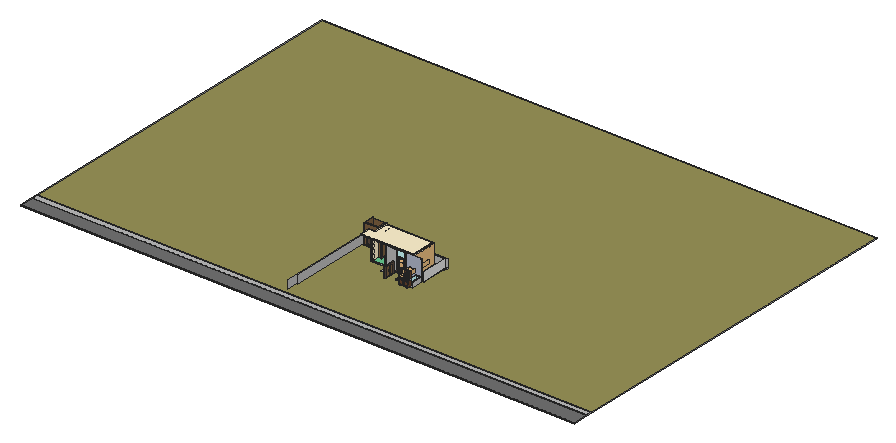
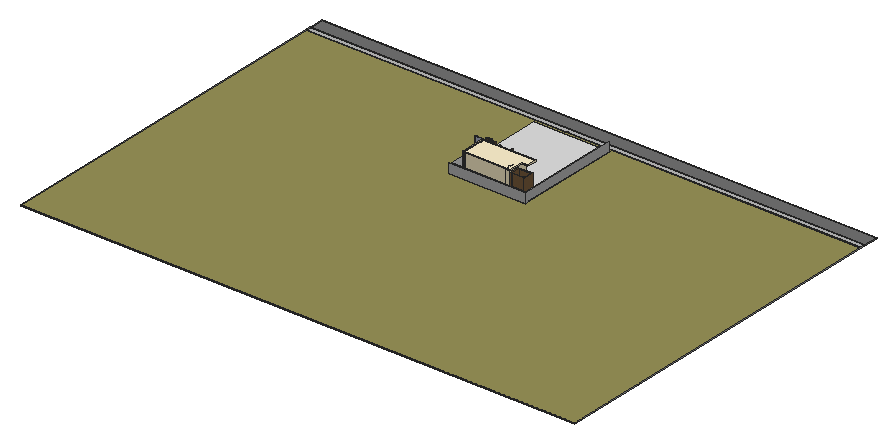
# SketchUp Ruby script. Lengths in inches.
U = 1.inch
M = Sketchup.active_model
def pt(a) = Geom::Point3d.new(a.map { |v| v * U })
def face(e, loops, mat)
  f = e.add_face(loops[0].map { |a| pt(a) })
  loops[1..].each { |l| e.add_face(l.map { |a| pt(a) }).erase! }
  f.material = f.back_material = mat if mat
  f
end
# faces: each face lists its corners as indices into pts; further lists are holes
def faces(e, pts, list, mat = nil) = list.each { |f| face(e, (f[0].is_a?(Array) ? f : [f]).map { |l| l.map { |i| pts[i] } }, mat) }
# xy, xz, yz: faces in a plane at the given z, y or x. An outline is a flat list of corners, or four numbers for a rectangle; further outlines are holes
def ring(l) = l.size == 4 ? [[l[0], l[1]], [l[2], l[1]], [l[2], l[3]], [l[0], l[3]]] : l.each_slice(2).to_a
def flat(e, list, mat, &to3) = list.each { |f| face(e, (f[0].is_a?(Array) ? f : [f]).map { |l| ring(l).map { |u, v| to3.(u, v) } }, mat) }
def xy(e, z, list, mat = nil) = flat(e, list, mat) { |x, y| [x, y, z] }
def xz(e, y, list, mat = nil) = flat(e, list, mat) { |x, z| [x, y, z] }
def yz(e, x, list, mat = nil) = flat(e, list, mat) { |y, z| [x, y, z] }
def lines(e, pts, list) = list.each { |a, b| e.add_line(pt(pts[a]), pt(pts[b])) }
# prism: a flat outline (further loops are holes) pulled along v
def prism(e, loops, v, mat = nil)
  f = face(e, loops, mat); d = Geom::Vector3d.new(v.map { |x| x * U })
  f.pushpull(f.normal.samedirection?(d) ? d.length : -d.length)
end
def box(e, o, s, mat = nil) = prism(e, [[o, [o[0] + s[0], o[1], o[2]], [o[0] + s[0], o[1] + s[1], o[2]], [o[0], o[1] + s[1], o[2]]]], [0, 0, s[2]], mat)
def at(x, y, z, deg = 0) = Geom::Transformation.translation(pt([x, y, z])) * Geom::Transformation.rotation(ORIGIN, Z_AXIS, deg.degrees)
def axes(o, x, y, z) = Geom::Transformation.new([*x, 0, *y, 0, *z, 0, *pt(o).to_a, 1])
def part(name) = M.definitions.add(name)
# library, detail: a bought-in or finely detailed component or shape, given as its bounding box
def library(name, o, s) = part(name).tap { |d| box(d.entities, o, s) }
def detail(e, o, s) = box(e.add_group.entities, o, s)
def put(e, d, t, mat = nil) = e.add_instance(d, t).tap { |i| i.material = mat if mat }
def group(e, t, mat = nil) = e.add_group.tap { |g| g.transformation = t; g.material = mat if mat }.entities
root = M.entities
M.materials.add("Brick_Stack_Bond_2K1").color = [104, 201, 144]
M.materials.add("Brick_Stack_Bond_2K2").color = [186, 186, 186]
M.materials.add("C02_Golden_Beige").color = [255, 205, 155]
M.materials.add("D01_Frost_White").color = [255, 242, 206]
M.materials.add("E03_Spring_Dew").color = [255, 255, 101]
M.materials.add("Glass_Sky Reflection_1").color = [126, 138, 183]
M.materials["Glass_Sky Reflection_1"].alpha = 0.25
M.materials.add("H01_Misty_Ice1").color = [204, 255, 255]
M.materials.add("M00_Soft_Cloud").color = [255, 255, 255]
M.materials.add("M01_Silver_Fog").color = [224, 224, 224]
M.materials.add("M02_Ash_Whisper").color = [196, 196, 196]
M.materials.add("M03_Pewter_Shine").color = [168, 168, 168]
M.materials.add("M05_Graphite_Haze").color = [114, 114, 114]
M.materials.add("M09_Shadow_Night").color = [0, 0, 0]
M.materials.add("Marble_03_1K").color = [175, 182, 201]
M.materials.add("Marble_07_1K").color = [36, 34, 36]
M.materials.add("Metal_06_1K").color = [238, 236, 231]
M.materials.add("Plaster_04_1K").color = [106, 98, 87]
M.materials.add("Plywood_01_1K").color = [125, 96, 64]
M.materials.add("Soil_04_1K").color = [167, 182, 67]
M.materials.add("Soil_04_1K1").color = [152, 146, 88]
M.materials.add("Wood_Floor_01_1K1").color = [146, 111, 76]
M.materials.add("Wood_Floor_12_1K").color = [92, 75, 65]
M.materials.add("Wood_Veneer_15_1K").color = [103, 69, 45]
c1 = part("Group\#174")
box(c1.entities,[0,0,0],[1.8125,10.875,0.375],"Metal_06_1K")
c2 = part("Shower Cabin 003")
xy(c2.entities,0,[[-0.1,-35.53,-0.1,-0.1,35.33,-35.53],[35.33,-35.53,-0.1,-0.1,35.33,-0.1]])
xy(c2.entities,0.39,[[2.26,-33.17,32.97,-2.46,2.26,-2.46],[2.26,-33.17,32.97,-33.17,32.97,-2.46]])
xy(c2.entities,1.18,[[-0.1,-35.53,1.48,-1.67,-0.1,-0.1],[-0.1,-35.53,1.48,-33.96,1.48,-1.67],[-0.1,-35.53,35.33,-35.53,1.48,-33.96],[35.33,-35.53,33.76,-33.96,1.48,-33.96],[35.33,-35.53,35.33,-0.1,33.76,-33.96],
  [33.76,-33.96,35.33,-0.1,33.76,-1.67],[1.48,-1.67,33.76,-1.67,-0.1,-0.1],[33.76,-1.67,35.33,-0.1,-0.1,-0.1]])
xz(c2.entities,-35.53,[[-0.1,0,35.33,0,35.33,1.18],[-0.1,0,35.33,1.18,-0.1,1.18]])
xz(c2.entities,-0.1,[[-0.1,0,-0.1,1.18,35.33,0],[35.33,0,-0.1,1.18,35.33,1.18]])
yz(c2.entities,-0.1,[[-0.1,0,-35.53,1.18,-0.1,1.18],[-35.53,0,-35.53,1.18,-0.1,0]])
yz(c2.entities,35.33,[[-35.53,0,-0.1,0,-0.1,1.18],[-35.53,0,-0.1,1.18,-35.53,1.18]])
p = [[1.48,-33.96,1.18],[2.26,-2.46,0.39],[1.48,-1.67,1.18],[33.76,-33.96,1.18],[2.26,-33.17,0.39],[32.97,-33.17,0.39],
  [33.76,-1.67,1.18],[32.97,-2.46,0.39]]
faces(c2.entities,p,[[0,1,2],[3,4,0],[0,4,1],[3,5,4],[6,5,3],[6,7,5],[2,7,6],[2,1,7]])
c3 = library("Hospital Sink 001",[-20.625,-17.4375,27.15],[31.24,200.7,22.96])
c4 = library("Group\#265",[0,0,0],[16.41,13,26.86])
c5 = library("Group\#200",[-159,9,0],[183,135,46])
c6 = library("Group\#210",[-7.75,0,-2.45],[16.75,48,50.51])
c7 = library("Group\#232",[-0.03,0,0],[10.08,153,132])
c8 = library("Group\#259",[0,0,0],[16.41,13,26.86])
xy(root,6,[[1567.75,149.6875,2047.75,798.625],[1567.75,798.625,1567.75,815.6875,2047.75,815.6875,2047.75,798.625,2044.5625,798.625,2044.5625,806.6875,1574.3125,806.6875,1574.3125,798.625]],"M01_Silver_Fog")
xy(root,12,[[1810.75,590.6875,1876.75,626.6875],[1926.75,626.6875,1939.75,635.6875],[1712.6875,635.6875,1721.6875,635.6875,1721.6875,779.6875,1977.9375,779.6875,1977.9375,635.6875,1986.9375,635.6875,1986.9375,788.6875,1712.6875,788.6875],[1721.6875,635.6875,1977.9375,779.6875]],"Brick_Stack_Bond_2K2")
xy(root,12,[[1886.75,626.6875,1926.75,635.6875]],"H01_Misty_Ice1")
xy(root,12,[[2044.5625,635.6875,2047.75,798.625],[1584.5,798.625,1674.5,806.6875]],"M01_Silver_Fog")
xy(root,12,[[1712.6875,635.6875,1986.9375,788.6875]],"M02_Ash_Whisper")
xy(root,12,[[1574.3125,798.625,1584.5,806.6875],[1674.5,798.625,2044.5625,806.6875]],"Soil_04_1K")
xy(root,18,[[1712.6875,635.6875,1942.625,635.6875,1942.625,671,1977.9375,671,1977.9375,635.6875,1986.9375,635.6875,1986.9375,788.6875,1712.6875,788.6875]],"Brick_Stack_Bond_2K1")
xy(root,18,[[1876.75,602.25,1882.75,626.6875],[1590.5,746.6875,1668.5,802.6875]],"Brick_Stack_Bond_2K2")
xy(root,18,[[1882.75,625.625,1886.75,626.6875],[1926.75,625.625,1930.75,626.6875],[1584.5,740.6875,1584.5,806.6875,1674.5,806.6875,1674.5,740.6875,1635.0625,740.6875,1635.0625,746.6875,1668.5,746.6875,1668.5,802.6875,1590.5,802.6875,1590.5,746.6875,1599.0625,746.6875,1599.0625,740.6875],[1599.0625,740.6875,1635.0625,746.6875]],"Plywood_01_1K")
xy(root,21.375,[[1942.625,635.6875,1977.9375,671]],"M02_Ash_Whisper")
xy(root,71.8125,[[1942.625,635.6875,1977.9375,671]],"M02_Ash_Whisper")
xy(root,73.25,[[1942.625,635.6875,1977.9375,671]],"M02_Ash_Whisper")
xy(root,99.75,[[1942.625,635.6875,1977.9375,671]],"M02_Ash_Whisper")
xy(root,100.8125,[[1942.625,635.6875,1977.9375,671]],"M00_Soft_Cloud")
xz(root,602.25,[[1876.75,18,1882.75,82.875]],"H01_Misty_Ice1")
xz(root,625.625,[[1882.75,18,1886.75,18,1886.75,99,1926.75,99,1926.75,18,1930.75,18,1930.75,103,1882.75,103]],"Plywood_01_1K")
xz(root,626.6875,[[1810.75,12,1876.75,139],[1926.75,12,1930.75,18],[1876.75,18,1882.75,144],[1882.75,18,1886.75,23],[1926.75,18,1930.75,103]],"Brick_Stack_Bond_2K2")
xz(root,626.6875,[[1876.75,12,1886.75,18],[1930.75,12,1939.75,12,1939.75,139,1882.75,139,1882.75,103,1930.75,103]],"H01_Misty_Ice1")
xz(root,635.6875,[[1986.9375,12,2044.5625,18],[2044.5625,12,2047.75,18]],"D01_Frost_White")
xz(root,635.6875,[[1810.75,12,1810.75,139,1939.75,139,1939.75,12,1926.75,12,1926.75,99,1886.75,99,1886.75,12],[1939.75,12,1977.9375,18],[1977.9375,12,1986.9375,18]],"H01_Misty_Ice1")
xz(root,635.6875,[[1942.625,21.375,1977.9375,71.8125],[1942.625,73.25,1977.9375,99.75]],"M00_Soft_Cloud")
xz(root,635.6875,[[2044.5625,18,2047.75,66]],"M01_Silver_Fog")
xz(root,635.6875,[[1712.6875,12,1986.9375,12,1986.9375,18,1977.9375,18,1977.9375,21.375,1942.625,21.375,1942.625,18,1712.6875,18],[1942.625,71.8125,1977.9375,73.25],[1942.625,99.75,1977.9375,100.8125]],"M02_Ash_Whisper")
xz(root,671,[[1942.625,21.375,1977.9375,71.8125],[1942.625,73.25,1977.9375,99.75]],"M00_Soft_Cloud")
xz(root,671,[[1942.625,18,1977.9375,21.375],[1942.625,71.8125,1977.9375,73.25],[1942.625,99.75,1977.9375,100.8125]],"M02_Ash_Whisper")
xz(root,740.6875,[[1584.5,12,1674.5,18],[1584.5,18,1599.0625,18,1599.0625,102,1635.0625,102,1635.0625,18,1674.5,18,1674.5,139,1584.5,139]],"Plywood_01_1K")
xz(root,746.6875,[[1590.5,18,1590.5,139,1668.5,139,1668.5,18,1635.0625,18,1635.0625,102,1599.0625,102,1599.0625,18]],"Plywood_01_1K")
xz(root,788.6875,[[1712.6875,12,1986.9375,18]],"M02_Ash_Whisper")
xz(root,798.625,[[1567.75,6,1574.3125,12],[1574.3125,6,2044.5625,12],[2044.5625,6,2047.75,12]],"M01_Silver_Fog")
xz(root,802.6875,[[1590.5,18,1668.5,139]],"Plywood_01_1K")
xz(root,806.6875,[[1674.5,12,2044.5625,66]],"Brick_Stack_Bond_2K2")
xz(root,806.6875,[[1574.3125,6,1584.5,12],[1584.5,6,1674.5,12],[1674.5,6,2044.5625,12]],"M01_Silver_Fog")
xz(root,806.6875,[[1574.3125,12,1584.5,66]],"M03_Pewter_Shine")
xz(root,806.6875,[[1584.5,12,1674.5,18],[1584.5,18,1674.5,66]],"Plywood_01_1K")
xz(root,815.6875,[[2047.75,0,2053.75,12],[1567.75,6,1567.75,66,2053.75,66,2053.75,12,2047.75,12,2047.75,6]],"Brick_Stack_Bond_2K2")
yz(root,1567.75,[[798.625,6,798.625,12,155.6875,12,155.6875,66,815.6875,66,815.6875,6]],"Brick_Stack_Bond_2K2")
yz(root,1574.3125,[[224.6875,12,806.6875,66]],"Brick_Stack_Bond_2K2")
yz(root,1574.3125,[[798.625,6,806.6875,12]],"M01_Silver_Fog")
yz(root,1584.5,[[740.6875,12,806.6875,18],[740.6875,18,806.6875,139]],"Plywood_01_1K")
yz(root,1590.5,[[746.6875,18,802.6875,139]],"Plywood_01_1K")
yz(root,1599.0625,[[740.6875,18,746.6875,102]],"Plywood_01_1K")
yz(root,1635.0625,[[740.6875,18,746.6875,102]],"Plywood_01_1K")
yz(root,1668.5,[[746.6875,18,802.6875,139]],"Plywood_01_1K")
yz(root,1674.5,[[740.6875,12,806.6875,18],[740.6875,18,806.6875,139]],"Plywood_01_1K")
yz(root,1712.6875,[[635.6875,12,788.6875,18]],"M02_Ash_Whisper")
yz(root,1810.75,[[626.6875,12,635.6875,139]],"Brick_Stack_Bond_2K2")
yz(root,1882.75,[[625.625,18,626.6875,23]],"Brick_Stack_Bond_2K2")
yz(root,1882.75,[[602.25,18,625.625,23]],"Wood_Floor_12_1K")
yz(root,1886.75,[[626.6875,12,635.6875,99]],"H01_Misty_Ice1")
yz(root,1886.75,[[625.625,18,626.6875,99]],"Plywood_01_1K")
yz(root,1926.75,[[626.6875,12,635.6875,99]],"H01_Misty_Ice1")
yz(root,1926.75,[[625.625,18,626.6875,99]],"Plywood_01_1K")
yz(root,1930.75,[[625.625,18,626.6875,103]],"Plywood_01_1K")
yz(root,1939.75,[[626.6875,12,635.6875,18]],"Brick_Stack_Bond_2K2")
yz(root,1939.75,[[626.6875,18,635.6875,139]],"H01_Misty_Ice1")
yz(root,1939.75,[[569.6875,12,626.6875,18]],"Marble_03_1K")
yz(root,1942.625,[[635.6875,21.375,671,71.8125],[635.6875,73.25,671,99.75]],"M00_Soft_Cloud")
yz(root,1942.625,[[635.6875,18,671,21.375],[635.6875,71.8125,671,73.25],[635.6875,99.75,671,100.8125]],"M02_Ash_Whisper")
yz(root,1977.9375,[[635.6875,18,671,21.375],[635.6875,21.375,671,71.8125]],"Brick_Stack_Bond_2K1")
yz(root,1977.9375,[[635.6875,71.8125,671,73.25],[635.6875,73.25,671,99.75],[635.6875,99.75,671,100.8125]],"M02_Ash_Whisper")
yz(root,1986.9375,[[635.6875,12,788.6875,18]],"M02_Ash_Whisper")
yz(root,2044.5625,[[798.625,6,806.6875,12],[635.6875,12,806.6875,66]],"M01_Silver_Fog")
p = [[1926.75,626.6875,18],[1886.75,626.6875,18]]
lines(root,p,[[0,1]])
g1 = group(root,at(1876.75,533.5,18),"Brick_Stack_Bond_2K2")
xy(g1,0,[[0,0,6,68.75]],"Wood_Floor_12_1K")
xy(g1,0.75,[[0,5.4375,4.5,34.21],[0,35.41,4.5,64.1875]])
xy(g1,0.75,[[4.5,5.4375,6,34.21],[0,34.21,6,35.41],[4.5,35.41,6,64.1875]],"Wood_Floor_12_1K")
xy(g1,59.875,[[0,5,4.5,34.21],[0,35.41,4.5,63.75]])
xy(g1,59.875,[[4.5,5,6,34.21],[0,34.21,6,35.41],[4.5,35.41,6,63.75]],"Wood_Floor_12_1K")
xy(g1,64.875,[[0,0,6,68.75]],"Wood_Floor_12_1K")
xz(g1,0,[[0,0,6,64.875]],"Wood_Floor_12_1K")
xz(g1,34.21,[[4.5,0.75,6,59.875]],"Wood_Floor_12_1K")
xz(g1,35.41,[[4.5,0.75,6,59.875]],"Wood_Floor_12_1K")
xz(g1,68.75,[[0,0,6,64.875]],"Wood_Floor_12_1K")
yz(g1,0,[[[0,0,68.75,64.875],[5.4375,0.75,64.1875,0.75,63.75,59.875,5,59.875]]],"Wood_Floor_12_1K")
yz(g1,4.5,[[5.4375,0.75,34.21,0.75,34.21,59.875,5,59.875],[35.41,0.75,64.1875,0.75,63.75,59.875,35.41,59.875]],"Plywood_01_1K")
yz(g1,6,[[[0,0,68.75,64.875],[5.4375,0.75,5,59.875,63.75,59.875,64.1875,0.75]],[34.21,0.75,35.41,59.875]],"Wood_Floor_12_1K")
p = [[0,5.4375,0.75],[0,5,59.875],[4.5,5,59.875],[4.5,5.4375,0.75],[6,5.4375,0.75],[6,5,59.875],
  [0,63.75,59.875],[0,64.1875,0.75],[4.5,64.1875,0.75],[4.5,63.75,59.875],[6,63.75,59.875],[6,64.1875,0.75]]
faces(g1,p,[[0,1,2,3],[6,7,8,9]])
faces(g1,p,[[4,3,2,5],[10,9,8,11]],"Wood_Floor_12_1K")
put(g1,c1,axes([4.5,28.44,28.59],[0,1,0],[0,0,1],[1,0,0]))
put(g1,c1,axes([4.5,38.94,28.59],[0,1,0],[0,0,1],[1,0,0]))
g2 = group(root,at(2002.95,558.2,18),"M02_Ash_Whisper")
p = [[35.375,-0.32,18.93],[0.01,-0.33,18.93],[0.01,0.17,-9.625],[35.375,0.17,-9.625],[0,67.67,20.12],[0,68.17,-8.44],
  [35.37,67.68,20.12],[35.37,68.17,-8.44],[2.68,64.99,20.07],[2.69,2.35,18.98],[2.69,2.68,0.17],[2.68,65.32,1.26],
  [32.69,2.36,18.98],[32.69,2.68,0.17],[32.68,64.99,20.07],[32.68,65.32,1.26]]
faces(g2,p,[[0,1,2,3],[1,4,5,2],[6,0,3,7],[7,3,2,5],[4,6,7,5],[[0,6,4,1],[9,8,14,12]]])
faces(g2,p,[[8,9,10,11],[9,12,13,10],[12,14,15,13],[11,10,13,15],[14,8,11,15]],"H01_Misty_Ice1")
put(root,c2,axes([1932.45,626.78,18],[1.99615,0,0],[0,1.9303,0],[0,0,1]),"M02_Ash_Whisper")
g3 = group(root,at(1939.75,626.6875,18),"M02_Ash_Whisper")
box(g3,[-8.0625,-0.5,0],[107.0625,0.5,126],"Marble_03_1K")
g4 = group(root,at(1969.5625,532.5625,18),"M02_Ash_Whisper")
put(g4,c3,at(16.5,21.23,2.77))
g5 = group(g4,at(0,21.52,36.9375),"Wood_Veneer_15_1K")
xy(g5,0,[[29.78,-9.4375,29.78,-0.9375,0,-0.9375,0,0,59.5625,0,59.5625,-9.4375]])
xy(g5,1,[[30.78,-9.4375,58.5625,-0.9375]])
xy(g5,16.65,[[30.78,-9.4375,58.5625,-0.9375]])
xy(g5,17.59,[[30.78,-9.4375,58.5625,-0.9375]])
xy(g5,31.28,[[30.78,-9.4375,58.5625,-0.9375]])
xy(g5,32.21,[[30.78,-9.4375,58.5625,-0.9375]])
xy(g5,44.5625,[[30.78,-9.4375,58.5625,-0.9375]])
xy(g5,45.5625,[[29.78,-9.4375,59.5625,-9.4375,59.5625,0,0,0,0,-0.9375,29.78,-0.9375]])
xz(g5,-9.4375,[[[29.78,0,59.5625,45.5625],[30.78,1,58.5625,16.65],[30.78,17.59,58.5625,31.28],[30.78,32.21,58.5625,44.5625]]])
xz(g5,-0.9375,[[0,0,29.78,45.5625],[30.78,1,58.5625,16.65],[30.78,17.59,58.5625,31.28],[30.78,32.21,58.5625,44.5625]])
xz(g5,0,[[0,0,59.5625,45.5625]])
yz(g5,0,[[-0.9375,0,0,45.5625]])
yz(g5,29.78,[[-9.4375,0,-0.9375,45.5625]])
yz(g5,30.78,[[-9.4375,1,-0.9375,16.65],[-9.4375,17.59,-0.9375,31.28],[-9.4375,32.21,-0.9375,44.5625]])
yz(g5,58.5625,[[-9.4375,1,-0.9375,16.65],[-9.4375,17.59,-0.9375,31.28],[-9.4375,32.21,-0.9375,44.5625]])
yz(g5,59.5625,[[-9.4375,0,0,45.5625]])
g6 = group(g5,at(6.54,-0.9375,15.81))
detail(g6,[0,-0.9375,-2.375],[14,0.9375,26.96])
g7 = group(g4,at(0,0.25,0),"Wood_Veneer_15_1K")
xy(g7,0,[[0,0,59.5625,21.4375]])
xy(g7,0,[[0,-0.25,59.5625,0]],"Wood_Floor_12_1K")
xy(g7,3,[[3,-0.25,28.78,0],[30.78,-0.25,56.5625,0]],"Wood_Floor_12_1K")
xy(g7,30.25,[[5.89,3.54,27.11,20.97]],"Marble_07_1K")
xy(g7,33,[[3,-0.25,28.78,0],[30.78,-0.25,56.5625,0]],"Wood_Floor_12_1K")
xy(g7,36,[[[0,0,59.5625,21.4375],[5.89,3.54,27.11,20.97]]],"Marble_07_1K")
xy(g7,36,[[0,-0.25,59.5625,0]],"Wood_Floor_12_1K")
xy(g7,36.9375,[[[0,0,59.5625,21.4375],[5.89,3.54,27.11,20.97]]],"Marble_03_1K")
xz(g7,-0.25,[[[0,0,59.5625,36],[3,3,28.78,33],[30.78,3,56.5625,33]]],"Wood_Floor_12_1K")
xz(g7,0,[[3,3,28.78,33],[30.78,3,56.5625,33]])
xz(g7,0,[[0,36,59.5625,36.9375]],"Marble_03_1K")
xz(g7,0,[[[0,0,59.5625,36],[3,3,28.78,33],[30.78,3,56.5625,33]]],"Wood_Floor_12_1K")
xz(g7,3.54,[[5.89,30.25,27.11,36],[5.89,36,27.11,36.9375]],"Marble_07_1K")
xz(g7,20.97,[[5.89,30.25,27.11,36],[5.89,36,27.11,36.9375]],"Marble_07_1K")
xz(g7,21.4375,[[0,0,59.5625,36]])
xz(g7,21.4375,[[0,36,59.5625,36.9375]],"Marble_07_1K")
yz(g7,0,[[0,0,21.4375,36]])
yz(g7,0,[[0,36,21.4375,36.9375]],"Marble_03_1K")
yz(g7,0,[[-0.25,0,0,36]],"Wood_Floor_12_1K")
yz(g7,3,[[-0.25,3,0,33]],"Wood_Floor_12_1K")
yz(g7,5.89,[[3.54,30.25,20.97,36],[3.54,36,20.97,36.9375]],"Marble_07_1K")
yz(g7,27.11,[[3.54,30.25,20.97,36],[3.54,36,20.97,36.9375]],"Marble_07_1K")
yz(g7,28.78,[[-0.25,3,0,33]],"Wood_Floor_12_1K")
yz(g7,30.78,[[-0.25,3,0,33]],"Wood_Floor_12_1K")
yz(g7,56.5625,[[-0.25,3,0,33]],"Wood_Floor_12_1K")
yz(g7,59.5625,[[0,0,21.4375,36]])
yz(g7,59.5625,[[0,36,21.4375,36.9375]],"Marble_03_1K")
yz(g7,59.5625,[[-0.25,0,0,36]],"Wood_Floor_12_1K")
put(root,c4,axes([1816.11,659.72,18],[1.29,0,0],[0,1.11,0],[0,0,1.58908]),"Wood_Floor_01_1K1")
put(root,c4,axes([1847,661.92,18],[1.29,0,0],[0,1.11,0],[0,0,1.58908]),"Wood_Floor_01_1K1")
put(root,c4,axes([1896.83,674.43,18],[0,1.29,0],[-1.11,0,0],[0,0,1.58908]),"Wood_Floor_01_1K1")
put(root,c4,axes([1796.42,701.64,18],[0,-1.29,0],[1.11,0,0],[0,0,1.58908]),"Wood_Floor_01_1K1")
g8 = group(root,at(1712.6875,635.6875,12),"Metal_06_1K")
xy(g8,51.49,[[265.25,55.375,274.25,103.375]],"H01_Misty_Ice1")
xy(g8,102,[[265.25,55.375,274.25,103.375]],"H01_Misty_Ice1")
xy(g8,126,[[-63.9375,0,-63.9375,63,-24.3125,63,-24.3125,153,0,153,0,0],[0,0,0,153,274.25,153,274.25,144,9,144,9,0],[9,0,265.25,9],[9,9,265.25,144]],"D01_Frost_White")
xy(g8,132,[[-63.9375,0,265.25,0,265.25,144,274.25,144,274.25,153,-24.3125,153,-24.3125,63,-63.9375,63],[265.25,0,274.25,144]],"D01_Frost_White")
xz(g8,0,[[0,0,9,126],[9,0,265.25,6],[265.25,0,274.25,132],[-63.9375,126,265.25,132]],"D01_Frost_White")
xz(g8,55.375,[[265.25,51.49,274.25,102]],"H01_Misty_Ice1")
xz(g8,63,[[-63.9375,126,-24.3125,132]],"D01_Frost_White")
xz(g8,103.375,[[265.25,51.49,274.25,102]],"H01_Misty_Ice1")
xz(g8,144,[[9,6,83.75,126],[83.75,6,265.25,126],[265.25,126,274.25,132]],"D01_Frost_White")
xz(g8,153,[[0,0,274.25,126],[-24.3125,126,274.25,132]],"D01_Frost_White")
yz(g8,-63.9375,[[0,126,63,132]],"D01_Frost_White")
yz(g8,-24.3125,[[63,126,153,132]],"D01_Frost_White")
yz(g8,0,[[0,0,153,126]],"D01_Frost_White")
yz(g8,9,[[0,6,9,126],[9,6,144,126]],"D01_Frost_White")
yz(g8,265.25,[[0,6,9,126]],"D01_Frost_White")
yz(g8,274.25,[[0,126,9,132],[9,126,144,132],[144,126,153,132]],"D01_Frost_White")
g9 = group(g8,at(229.9375,0,6))
xy(g9,0,[[0,0,35.3125,35.3125]])
put(g8,c5,at(241.25,0,6))
put(g8,c6,at(265.25,55.375,53.9375),"C02_Golden_Beige")
g10 = group(g8,at(264.68,127.41,101.75),"M09_Shadow_Night")
box(g10,[-0.5,0,0],[0.5,1.4375,8.5625])
g11 = group(g8,at(264.93,123.12,91.45))
yz(g11,-0.75,[[4.72,0,3.39,0.29,2.19,0.92,1.19,1.83,0.47,2.98,0.06,4.27,0,5.62,0.29,6.94,0.92,8.14,1.83,9.14,2.98,9.87,4.27,10.28,5.62,10.34,6.94,10.04,8.14,9.42,9.14,8.5,9.87,7.36,10.28,6.07,10.34,4.72,10.04,3.39,9.42,2.19,8.5,1.19,7.36,0.47,6.07,0.06]],"M09_Shadow_Night")
yz(g11,0,[[4.72,0,6.07,0.06,7.36,0.47,8.5,1.19,9.42,2.19,10.04,3.39,10.34,4.72,10.28,6.07,9.87,7.36,9.14,8.5,8.14,9.42,6.94,10.04,5.62,10.34,4.27,10.28,2.98,9.87,1.83,9.14,0.92,8.14,0.29,6.94,0,5.62,0.06,4.27,0.47,2.98,1.19,1.83,2.19,0.92,3.39,0.29]])
p = [[0,4.72,0],[0,3.39,0.29],[-0.75,3.39,0.29],[-0.75,4.72,0],[0,6.07,0.06],[-0.75,6.07,0.06],
  [0,7.36,0.47],[-0.75,7.36,0.47],[0,2.19,0.92],[-0.75,2.19,0.92],[0,8.5,1.19],[-0.75,8.5,1.19],
  [0,1.19,1.83],[-0.75,1.19,1.83],[0,9.42,2.19],[-0.75,9.42,2.19],[0,0.47,2.98],[-0.75,0.47,2.98],
  [0,10.04,3.39],[-0.75,10.04,3.39],[0,0.06,4.27],[-0.75,0.06,4.27],[0,10.34,4.72],[-0.75,10.34,4.72],
  [0,0,5.62],[-0.75,0,5.62],[0,10.28,6.07],[-0.75,10.28,6.07],[0,0.29,6.94],[-0.75,0.29,6.94],
  [0,9.87,7.36],[-0.75,9.87,7.36],[0,0.92,8.14],[-0.75,0.92,8.14],[0,9.14,8.5],[-0.75,9.14,8.5],
  [0,1.83,9.14],[-0.75,1.83,9.14],[0,8.14,9.42],[-0.75,8.14,9.42],[0,2.98,9.87],[-0.75,2.98,9.87],
  [0,6.94,10.04],[-0.75,6.94,10.04],[0,4.27,10.28],[-0.75,4.27,10.28],[0,5.62,10.34],[-0.75,5.62,10.34]]
faces(g11,p,[[0,1,2,3],[4,0,3,5],[6,4,5,7],[1,8,9,2],[10,6,7,11],[8,12,13,9],[14,10,11,15],[12,16,17,13],
  [18,14,15,19],[16,20,21,17],[22,18,19,23],[20,24,25,21],[26,22,23,27],[24,28,29,25],[30,26,27,31],[28,32,33,29],
  [34,30,31,35],[32,36,37,33],[38,34,35,39],[36,40,41,37],[42,38,39,43],[40,44,45,41],[46,42,43,47],[44,46,47,45]],"M09_Shadow_Night")
g12 = group(g8,at(264.68,119.33,94.55))
xy(g12,-5.125,[[-0.4375,-2.75,0,3.3125]],"E03_Spring_Dew")
xy(g12,0,[[-0.4375,-2.75,0,0],[-0.4375,0,0,0.8125],[-0.4375,0.8125,0,3.3125]],"E03_Spring_Dew")
xy(g12,6.0625,[[-0.4375,0,0,0.8125]],"E03_Spring_Dew")
xz(g12,-2.75,[[-0.4375,-5.125,0,0]],"E03_Spring_Dew")
xz(g12,0,[[-0.4375,0,0,6.0625]],"E03_Spring_Dew")
xz(g12,0.8125,[[-0.4375,0,0,6.0625]],"E03_Spring_Dew")
xz(g12,3.3125,[[-0.4375,-5.125,0,0]],"E03_Spring_Dew")
yz(g12,-0.4375,[[-2.75,-5.125,3.3125,0],[0,0,0.8125,6.0625]],"E03_Spring_Dew")
yz(g12,0,[[-2.75,-5.125,3.3125,0],[0,0,0.8125,6.0625]],"E03_Spring_Dew")
g13 = group(g8,at(264.68,121.99,100.65))
xy(g13,0,[[-0.375,0,0,0.09],[-0.375,0.09,0,0.11]],"Metal_06_1K")
xy(g13,11.74,[[-0.375,0,0,0.11]],"Metal_06_1K")
xz(g13,0,[[-0.375,0,0,11.74]],"Metal_06_1K")
xz(g13,0.11,[[-0.375,0,0,11.74]],"Metal_06_1K")
xz(g13,1.72,[[-0.375,-1.24,-0.125,-0.85],[-0.125,-1.24,0,-0.85]],"Metal_06_1K")
yz(g13,-0.375,[[0.09,-2.09,-0.34,-2.06,-0.74,-1.95,-1.08,-1.79,-1.35,-1.57,-1.51,-1.32,-1.57,-1.05,-1.51,-0.78,-1.35,-0.52,-1.08,-0.31,-0.74,-0.14,-0.34,-0.04,0.09,0,0.52,-0.04,0.92,-0.14,1.27,-0.31,1.53,-0.52,1.7,-0.78,1.72,-0.85,1.72,-1.24,1.7,-1.32,1.53,-1.57,1.27,-1.79,0.92,-1.95,0.52,-2.06],[0,0,0.11,11.74]],"Metal_06_1K")
yz(g13,-0.125,[[1.72,-1.24,1.72,-0.85,1.76,-1.05]])
yz(g13,0,[[0.09,-2.09,0.52,-2.06,0.92,-1.95,1.27,-1.79,1.53,-1.57,1.7,-1.32,1.72,-1.24,1.72,-0.85,1.7,-0.78,1.53,-0.52,1.27,-0.31,0.92,-0.14,0.52,-0.04,0.09,0,-0.34,-0.04,-0.74,-0.14,-1.08,-0.31,-1.35,-0.52,-1.51,-0.78,-1.57,-1.05,-1.51,-1.32,-1.35,-1.57,-1.08,-1.79,-0.74,-1.95,-0.34,-2.06],[0,0,0.11,11.74]],"Metal_06_1K")
p = [[0,-0.74,-1.95],[-0.375,-0.74,-1.95],[-0.375,-0.34,-2.06],[0,-0.34,-2.06],[-0.375,0.09,-2.09],[0,0.09,-2.09],
  [-0.375,0.52,-2.06],[0,0.52,-2.06],[-0.375,0.92,-1.95],[0,0.92,-1.95],[0,-1.08,-1.79],[-0.375,-1.08,-1.79],
  [-0.375,1.27,-1.79],[0,1.27,-1.79],[0,-1.35,-1.57],[-0.375,-1.35,-1.57],[-0.375,1.53,-1.57],[0,1.53,-1.57],
  [0,-1.51,-1.32],[-0.375,-1.51,-1.32],[-0.375,1.7,-1.32],[0,1.7,-1.32],[0,-1.57,-1.05],[-0.375,-1.57,-1.05],
  [-0.375,1.72,-1.24],[-0.125,1.72,-1.24],[0,1.72,-1.24],[0,-1.51,-0.78],[-0.375,-1.51,-0.78],[0,1.72,-0.85],
  [-0.125,1.72,-0.85],[-0.375,1.72,-0.85],[-0.375,1.7,-0.78],[0,1.7,-0.78],[0,-1.35,-0.52],[-0.375,-1.35,-0.52],
  [-0.375,1.53,-0.52],[0,1.53,-0.52],[0,-1.08,-0.31],[-0.375,-1.08,-0.31],[-0.375,1.27,-0.31],[0,1.27,-0.31],
  [0,-0.74,-0.14],[-0.375,-0.74,-0.14],[-0.375,0.92,-0.14],[0,0.92,-0.14],[0,-0.34,-0.04],[-0.375,-0.34,-0.04],
  [-0.375,0.52,-0.04],[0,0.52,-0.04],[0,0.09,0],[-0.375,0.09,0]]
faces(g13,p,[[0,1,2,3],[3,2,4,5],[5,4,6,7],[7,6,8,9],[10,11,1,0],[9,8,12,13],[14,15,11,10],[13,12,16,17],
  [18,19,15,14],[17,16,20,21],[22,23,19,18],[21,20,24,25,26],[27,28,23,22],[29,30,31,32,33],[34,35,28,27],[33,32,36,37],
  [38,39,35,34],[37,36,40,41],[42,43,39,38],[41,40,44,45],[46,47,43,42],[45,44,48,49],[50,51,47,46],[49,48,51,50]],"Metal_06_1K")
put(g8,c7,axes([264.2,0,0],[1,0,0],[0,1,0],[0,0,0.95455]),"D01_Frost_White")
put(root,c8,axes([1868.33,719.79,18],[-1.29,0,0],[0,-1.11,0],[0,0,1.58908]),"Wood_Floor_01_1K1")
put(root,c4,axes([1836.83,719.79,18],[-1.29,0,0],[0,-1.11,0],[0,0,1.58908]),"Wood_Floor_01_1K1")
g14 = group(root,at(1721.6875,662.1875,18),"M02_Ash_Whisper")
xy(g14,0,[[0,16.6875,20.5,117.5],[20.5,16.6875,21.5,117.5]],"Plywood_01_1K")
xy(g14,2.61,[[7.625,68.09,20.5,90.3],[7.625,92.3,20.5,114.5]],"Plywood_01_1K")
xy(g14,2.61,[[20.5,19.6875,21.5,66.09],[20.5,68.09,21.5,90.3],[20.5,92.3,21.5,114.5]],"Wood_Floor_12_1K")
xy(g14,39.45,[[7.625,68.09,20.5,90.3],[7.625,92.3,20.5,114.5]],"Plywood_01_1K")
xy(g14,39.45,[[20.5,68.09,21.5,90.3],[20.5,92.3,21.5,114.5]],"Wood_Floor_12_1K")
xy(g14,41.46,[[5.375,91.3,20.5,114.5]],"Plywood_01_1K")
xy(g14,41.46,[[20.5,68.09,21.5,114.5]],"Wood_Floor_12_1K")
xy(g14,49.74,[[5.375,91.3,20.5,114.5]],"Plywood_01_1K")
xy(g14,50.56,[[5.375,91.3,20.5,114.5]],"Plywood_01_1K")
xy(g14,62.46,[[5.375,91.3,20.5,114.5]],"Plywood_01_1K")
xy(g14,63.28,[[5.375,91.3,20.5,114.5]],"Plywood_01_1K")
xy(g14,74.24,[[20.5,68.09,21.5,114.5],[5.375,91.3,20.5,114.5]],"Plywood_01_1K")
xy(g14,75.77,[[20.5,68.09,21.5,114.5]],"Wood_Floor_12_1K")
xy(g14,107.01,[[20.5,19.6875,21.5,66.09],[20.5,68.09,21.5,114.5]],"Plywood_01_1K")
xy(g14,109.62,[[0,16.6875,20.5,117.5]],"Plywood_01_1K")
xy(g14,109.62,[[20.5,16.6875,21.5,117.5]],"Wood_Floor_12_1K")
xz(g14,16.6875,[[0,0,20.5,109.62]],"Plywood_01_1K")
xz(g14,16.6875,[[20.5,0,21.5,109.62]],"Wood_Floor_12_1K")
xz(g14,19.6875,[[20.5,2.61,21.5,107.01]],"Wood_Floor_12_1K")
xz(g14,66.09,[[20.5,2.61,21.5,107.01]],"Wood_Floor_12_1K")
xz(g14,68.09,[[7.625,2.61,20.5,39.45]],"Plywood_01_1K")
xz(g14,68.09,[[20.5,2.61,21.5,39.45],[20.5,41.46,21.5,74.24],[20.5,75.77,21.5,107.01]],"Wood_Floor_12_1K")
xz(g14,90.3,[[7.625,2.61,20.5,39.45]],"Plywood_01_1K")
xz(g14,90.3,[[20.5,2.61,21.5,39.45]],"Wood_Floor_12_1K")
xz(g14,91.3,[[5.375,41.46,20.5,49.74],[5.375,50.56,20.5,62.46],[5.375,63.28,20.5,74.24]],"Plywood_01_1K")
xz(g14,92.3,[[7.625,2.61,20.5,39.45]],"Plywood_01_1K")
xz(g14,92.3,[[20.5,2.61,21.5,39.45]],"Wood_Floor_12_1K")
xz(g14,114.5,[[7.625,2.61,20.5,39.45],[5.375,41.46,20.5,49.74],[5.375,50.56,20.5,62.46],[5.375,63.28,20.5,74.24]],"Plywood_01_1K")
xz(g14,114.5,[[20.5,2.61,21.5,39.45],[20.5,41.46,21.5,74.24],[20.5,75.77,21.5,107.01]],"Wood_Floor_12_1K")
xz(g14,117.5,[[0,0,20.5,109.62],[20.5,0,21.5,109.62]],"Plywood_01_1K")
yz(g14,0,[[16.6875,0,117.5,109.62]],"Plywood_01_1K")
yz(g14,5.375,[[91.3,41.46,114.5,49.74],[91.3,50.56,114.5,62.46],[91.3,63.28,114.5,74.24]],"Plywood_01_1K")
yz(g14,7.625,[[68.09,2.61,90.3,39.45],[92.3,2.61,114.5,39.45]],"Plywood_01_1K")
yz(g14,20.5,[[68.09,2.61,90.3,39.45],[92.3,2.61,114.5,39.45]],"Glass_Sky Reflection_1")
yz(g14,20.5,[[[16.6875,0,117.5,109.62],[19.6875,2.61,66.09,107.01],[68.09,41.46,114.5,74.24],[68.09,75.77,114.5,107.01],[92.3,2.61,114.5,39.45],[68.09,2.61,90.3,39.45]],[19.6875,2.61,66.09,107.01],[68.09,41.46,90.3,74.24],[91.3,49.74,114.5,50.56],[91.3,62.46,114.5,63.28],
  [68.09,75.77,114.5,107.01]],"Plywood_01_1K")
yz(g14,20.5,[[90.3,41.46,91.3,74.24]],"Wood_Floor_12_1K")
yz(g14,21.5,[[[16.6875,0,117.5,109.62],[19.6875,2.61,66.09,107.01],[68.09,41.46,114.5,74.24],[68.09,75.77,114.5,107.01],[92.3,2.61,114.5,39.45],[68.09,2.61,90.3,39.45]]],"Wood_Floor_12_1K")
g15 = group(g14,at(20.5,57.41,56.83))
box(g15,[0,0,0],[0.5625,2.0625,8.97],"Metal_06_1K")
g16 = group(root,at(1599.0625,746.6875,18),"Brick_Stack_Bond_2K2")
xy(g16,0,[[0,-6,36,0]],"Wood_Floor_12_1K")
xy(g16,3,[[3,-6,33,-4.75],[3,-4.75,33,0]],"Wood_Floor_12_1K")
xy(g16,81,[[3,-6,33,-4.75],[3,-4.75,33,0]],"Wood_Floor_12_1K")
xy(g16,84,[[0,-6,36,0]],"Wood_Floor_12_1K")
xz(g16,-6,[[[0,0,36,84],[3,3,33,81]]],"Wood_Floor_12_1K")
xz(g16,-4.75,[[3,3,33,81]],"Wood_Floor_12_1K")
xz(g16,0,[[[0,0,36,84],[3,3,33,81]]],"Wood_Floor_12_1K")
yz(g16,0,[[-6,0,0,84]],"Wood_Floor_12_1K")
yz(g16,3,[[-6,3,-4.75,81],[-4.75,3,0,81]],"Wood_Floor_12_1K")
yz(g16,33,[[-6,3,-4.75,81],[-4.75,3,0,81]],"Wood_Floor_12_1K")
yz(g16,36,[[-6,0,0,84]],"Wood_Floor_12_1K")
g17 = group(root,at(1567.75,215.6875,0),"M03_Pewter_Shine")
xy(g17,0,[[-1567.75,-121.25,1941.25,2172.3125]])
xy(g17,0,[[-1567.75,-215.6875,1941.25,-121.25]],"M02_Ash_Whisper")
xy(g17,6,[[-1567.75,-215.6875,1941.25,-121.25]],"M05_Graphite_Haze")
xy(g17,6,[[-1567.75,-86.0625,1941.25,2172.3125]],"Soil_04_1K1")
xy(g17,7.5,[[-1567.75,-121.25,1941.25,-86.0625]],"Brick_Stack_Bond_2K2")
xz(g17,-215.6875,[[-1567.75,0,1941.25,6]],"M05_Graphite_Haze")
xz(g17,-121.25,[[-1567.75,6,1941.25,7.5]],"M00_Soft_Cloud")
xz(g17,-121.25,[[-1567.75,0,1941.25,6]],"M02_Ash_Whisper")
xz(g17,-86.0625,[[-1567.75,6,294.07,7.5],[294.07,6,1941.25,7.5]],"Plaster_04_1K")
xz(g17,2172.3125,[[-1567.75,0,1941.25,6]])
yz(g17,-1567.75,[[-121.25,0,-121.25,7.5,-86.0625,7.5,-86.0625,6,2172.3125,6,2172.3125,0]])
yz(g17,-1567.75,[[-215.6875,0,-121.25,6]],"M05_Graphite_Haze")
yz(g17,1941.25,[[-121.25,0,2172.3125,0,2172.3125,6,-86.0625,6,-86.0625,7.5,-121.25,7.5]])
yz(g17,1941.25,[[-215.6875,0,-121.25,6]],"M05_Graphite_Haze")
